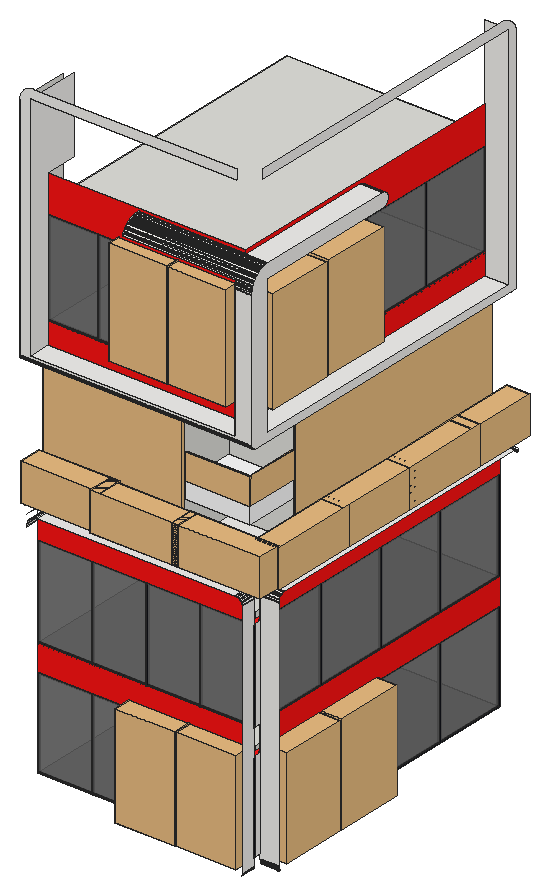
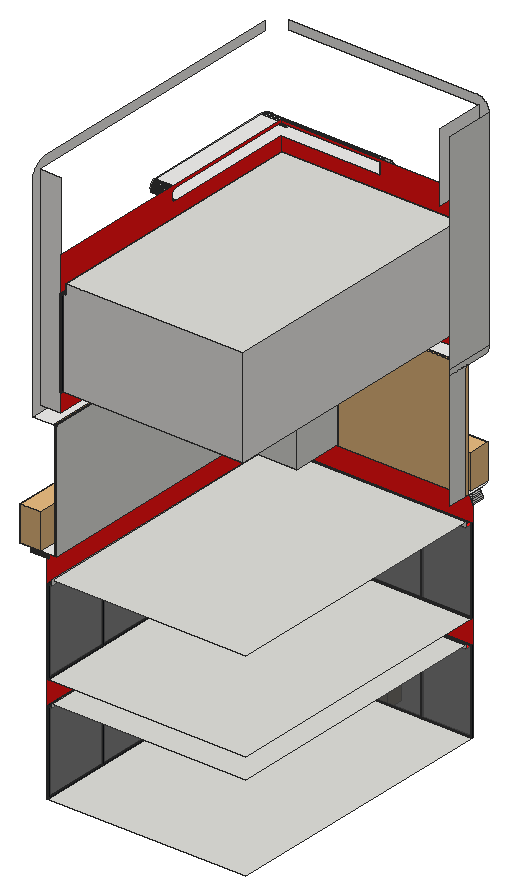
# SketchUp Ruby script. Lengths in inches.
U = 1.inch
M = Sketchup.active_model
def pt(a) = Geom::Point3d.new(a.map { |v| v * U })
def face(e, loops, mat)
  f = e.add_face(loops[0].map { |a| pt(a) })
  loops[1..].each { |l| e.add_face(l.map { |a| pt(a) }).erase! }
  f.material = f.back_material = mat if mat
  f
end
# faces: each face lists its corners as indices into pts; further lists are holes
def faces(e, pts, list, mat = nil) = list.each { |f| face(e, (f[0].is_a?(Array) ? f : [f]).map { |l| l.map { |i| pts[i] } }, mat) }
# xy, xz, yz: faces in a plane at the given z, y or x. An outline is a flat list of corners, or four numbers for a rectangle; further outlines are holes
def ring(l) = l.size == 4 ? [[l[0], l[1]], [l[2], l[1]], [l[2], l[3]], [l[0], l[3]]] : l.each_slice(2).to_a
def flat(e, list, mat, &to3) = list.each { |f| face(e, (f[0].is_a?(Array) ? f : [f]).map { |l| ring(l).map { |u, v| to3.(u, v) } }, mat) }
def xy(e, z, list, mat = nil) = flat(e, list, mat) { |x, y| [x, y, z] }
def xz(e, y, list, mat = nil) = flat(e, list, mat) { |x, z| [x, y, z] }
def yz(e, x, list, mat = nil) = flat(e, list, mat) { |y, z| [x, y, z] }
def lines(e, pts, list) = list.each { |a, b| e.add_line(pt(pts[a]), pt(pts[b])) }
# prism: a flat outline (further loops are holes) pulled along v
def prism(e, loops, v, mat = nil)
  f = face(e, loops, mat); d = Geom::Vector3d.new(v.map { |x| x * U })
  f.pushpull(f.normal.samedirection?(d) ? d.length : -d.length)
end
def box(e, o, s, mat = nil) = prism(e, [[o, [o[0] + s[0], o[1], o[2]], [o[0] + s[0], o[1] + s[1], o[2]], [o[0], o[1] + s[1], o[2]]]], [0, 0, s[2]], mat)
def at(x, y, z, deg = 0) = Geom::Transformation.translation(pt([x, y, z])) * Geom::Transformation.rotation(ORIGIN, Z_AXIS, deg.degrees)
def axes(o, x, y, z) = Geom::Transformation.new([*x, 0, *y, 0, *z, 0, *pt(o).to_a, 1])
def part(name) = M.definitions.add(name)
# library, detail: a bought-in or finely detailed component or shape, given as its bounding box
def library(name, o, s) = part(name).tap { |d| box(d.entities, o, s) }
def detail(e, o, s) = box(e.add_group.entities, o, s)
def put(e, d, t, mat = nil) = e.add_instance(d, t).tap { |i| i.material = mat if mat }
def group(e, t, mat = nil) = e.add_group.tap { |g| g.transformation = t; g.material = mat if mat }.entities
root = M.entities
M.materials.add("Generic").color = [242, 241, 238]
M.materials.add("Heather_Band").color = [255, 20, 20]
M.materials.add("[Color M00]").color = [255, 255, 255]
M.materials.add("{045efeae-c101-a24d-bd9b-6f5600100adb}").color = [102, 102, 102]
M.materials["{045efeae-c101-a24d-bd9b-6f5600100adb}"].alpha = 0.7
M.materials.add("{16756a1b-d383-d94f-ad82-104813d2624f}").color = [19, 21, 27]
c1 = library("Shrub+_Grass",[-121.83,-22.34,0],[123.96,19.94,123.95])
c2 = part("Furniture_0DcpanrIvuI8n_9Ae92L5A")
g1 = group(c2.entities,at(0,0,0))
box(g1,[-19.29,-0.2,0.39],[38.58,0.4,83.86],"{045efeae-c101-a24d-bd9b-6f5600100adb}")
g2 = group(c2.entities,at(0,0,0))
box(g2,[-19.68,-0.59,63.39],[39.36,1.18,0.39],"{16756a1b-d383-d94f-ad82-104813d2624f}")
box(g2,[-19.68,-0.59,42.52],[39.36,1.18,0.39],"{16756a1b-d383-d94f-ad82-104813d2624f}")
box(g2,[-19.68,-0.59,21.26],[39.36,1.18,0.39],"{16756a1b-d383-d94f-ad82-104813d2624f}")
xy(g2,0,[[-19.68,-0.59,19.68,0.59]],"{16756a1b-d383-d94f-ad82-104813d2624f}")
xy(g2,0.39,[[-19.68,-0.59,-19.29,0.59],[-19.68,-0.59,19.68,0.59],[19.29,-0.59,19.68,0.59]],"{16756a1b-d383-d94f-ad82-104813d2624f}")
xy(g2,84.25,[[-19.68,-0.59,19.68,0.59]],"{16756a1b-d383-d94f-ad82-104813d2624f}")
xy(g2,84.65,[[-19.68,-0.59,-19.29,0.59],[-19.68,-0.59,19.68,0.59],[19.29,-0.59,19.68,0.59]],"{16756a1b-d383-d94f-ad82-104813d2624f}")
xz(g2,-0.59,[[-19.68,0,19.68,0.39],[-19.68,0.39,-19.29,84.65],[19.29,0.39,19.68,84.65],[-19.68,84.25,19.68,84.65]],"{16756a1b-d383-d94f-ad82-104813d2624f}")
xz(g2,0.59,[[-19.68,0,19.68,0.39],[-19.68,0.39,-19.29,84.65],[19.29,0.39,19.68,84.65],[-19.68,84.25,19.68,84.65]],"{16756a1b-d383-d94f-ad82-104813d2624f}")
yz(g2,-19.68,[[-0.59,0,0.59,0.39],[-0.59,0.39,0.59,84.65],[-0.59,84.25,0.59,84.65]],"{16756a1b-d383-d94f-ad82-104813d2624f}")
yz(g2,-19.29,[[-0.59,0.39,0.59,84.65]],"{16756a1b-d383-d94f-ad82-104813d2624f}")
yz(g2,19.29,[[-0.59,0.39,0.59,84.65]],"{16756a1b-d383-d94f-ad82-104813d2624f}")
yz(g2,19.68,[[-0.59,0,0.59,0.39],[-0.59,0.39,0.59,84.65],[-0.59,84.25,0.59,84.65]],"{16756a1b-d383-d94f-ad82-104813d2624f}")
c3 = part("Glass+Window")
put(c3.entities,c2,at(0,0,-42.32))
c4 = library("Back Drop",[0,0,0],[82.68,2.27,107.48])
c5 = library("Planted timber trough",[0,0,0],[56.02,15.3,25.28])
c6 = library("My+Glass_Railing",[-0.07,0,0],[101.37,2.52,40.9])
c7 = library("My+Glass_Railing\#1",[-0.0625,0,0],[98.32,2.52,40.9])
xy(root,452.24,[[145.77,137.375,482.71,617.58]])
xy(root,592.96,[[145.77,137.375,145.77,151.79,474.55,151.79,474.55,617.58,482.71,617.58,482.71,137.375]],"Heather_Band")
xy(root,599,[[145.77,151.79,474.55,617.58]])
xy(root,633.64,[[145.77,137.375,482.71,617.58]])
xy(root,777.77,[[145.77,137.375,145.77,151.79,474.55,151.79,474.55,617.58,482.71,617.58,482.71,137.375]],"Heather_Band")
xy(root,786.62,[[145.77,151.79,474.55,617.58]])
xy(root,823.39,[[480.21,611.74,482.71,617.58]])
xy(root,823.39,[[164.14,115.9,470.91,137.375],[482.71,163.53,510.83,611.74]],"Generic")
xy(root,835.52,[[144.5,115.9,492.12,115.9,494.5625,116.0625,496.96,116.54,499.28,117.33,501.48,118.41,503.51,119.77,505.35,121.38,506.97,123.22,508.33,125.26,509.41,127.45,510.2,129.77,510.67,132.17,510.83,134.62,510.83,624.64,510.77,625.65,510.57,626.63,510.25,627.59,509.8,628.49,509.24,629.33,508.58,630.08,507.82,630.75,506.98,631.31,506.08,631.75,505.13,632.08,504.14,632.27,503.14,632.34,454.94,632.34,454.94,249.57,353.58,249.57,353.58,164.53,133.86,164.53,133.86,126.54,133.95,125.15,134.22,123.79,134.67,122.47,135.28,121.22,136.06,120.0625,136.98,119.02,138.02,118.1,139.18,117.33,140.43,116.71,141.75,116.26,143.11,115.99]],"Generic")
xy(root,895.84,[[353.58,164.53,454.94,249.57]],"[Color M00]")
xy(root,921.04,[[353.58,164.53,454.94,164.53,454.94,249.57,449.01,249.57,449.01,170.19,353.58,170.19]],"Generic")
xy(root,921.04,[[353.58,170.19,449.01,249.57]],"[Color M00]")
xy(root,1033.75,[[133.86,124.82,133.86,164.53,353.58,164.53,353.58,249.57,454.94,249.57,454.94,632.34,486.44,632.34,487.65,632.26,488.84,632.02,489.98,631.63,491.07,631.1,492.08,630.43,492.99,629.625,493.79,628.72,494.46,627.71,495,626.62,495.38,625.48,495.62,624.29,495.7,623.08,495.7,124.82],[495.7,623.08,495.62,624.29,495.38,625.48,495,626.62,494.46,627.71,493.79,628.72,492.99,629.625,492.08,630.43,491.07,631.1,489.98,631.63,488.84,632.02,487.65,632.26,486.44,632.34,495.7,632.34]],"Generic")
xy(root,1045.51,[[150.95,118.26,469.09,118.26,469.09,128.11,487.7,128.11,487.7,146.81,495.7,146.81,495.7,617.58,459.56,617.58,459.56,151.96,150.95,151.96]],"Generic")
xy(root,1078.9375,[[150.95,151.96,459.56,617.58]])
xy(root,1227.79,[[150.95,151.96,150.95,160.3,451.22,160.3,451.22,617.58,459.56,617.58,459.56,151.96]],"Heather_Band")
xy(root,1245.125,[[150.95,160.3,451.22,617.58]])
xy(root,1261.55,[[291.94,120.41,291.94,151.96,459.56,151.96,459.56,372.87,495.7,372.87,495.7,146.81,487.7,146.81,487.7,128.11,469.09,128.11,469.09,120.41]],"Generic")
xy(root,1281.6,[[291.94,149.74,495.7,149.74,495.7,372.87,459.56,372.87,459.56,151.96,291.94,151.96]],"Generic")
xz(root,118.26,[[133.86,1040.31,495.7,1040.31,495.7,1250.12,469.09,1250.12,469.09,1045.51,150.95,1045.51,150.95,1403.29,472.44,1403.29,472.44,1418.32,155.71,1418.32,154.28,1418.27,152.86,1418.13,151.45,1417.9,150.06,1417.57,148.6875,1417.16,147.35,1416.65,146.05,1416.0625,144.79,1415.39,143.57,1414.63,142.41,1413.8,141.3,1412.89,140.26,1411.92,139.28,1410.875,138.375,1409.77,137.54,1408.61,136.79,1407.39,136.11,1406.13,135.52,1404.83,135.02,1403.49,134.6,1402.12,134.28,1400.73,134.05,1399.32,133.91,1397.89,133.86,1396.46]],"Generic")
xz(root,128.11,[[469.09,1045.51,487.7,1261.55]])
xz(root,137.375,[[145.77,592.96,482.71,633.64],[145.77,777.77,482.71,777.77,482.71,812.85,482.46,814.27,482.04,815.65,481.46,816.97,480.72,818.21,479.84,819.35,478.82,820.37,477.69,821.27,476.46,822.02,475.14,822.61,473.77,823.04,472.35,823.3,470.91,823.39,164.14,823.39,161.74,823.23,159.38,822.77,157.11,821.99,154.95,820.93,152.95,819.6,151.15,818.01,149.5625,816.21,148.23,814.21,147.17,812.05,146.39,809.78,145.93,807.42,145.77,805.02]],"Heather_Band")
xz(root,146.81,[[487.7,1045.51,495.7,1261.55]])
xz(root,150.43,[[482.71,444.64,510.83,812.2]],"Generic")
xz(root,151.79,[[145.77,592.96,474.55,599],[145.77,777.77,474.55,786.62]])
xz(root,151.96,[[150.95,1045.51,459.56,1078.9375],[150.95,1227.79,459.56,1227.79,459.56,1261.55,291.94,1261.55,291.94,1281.6,459.56,1281.6,459.56,1286.04,150.95,1286.04]],"Heather_Band")
xz(root,160.3,[[150.95,1227.79,451.22,1245.125]])
xz(root,164.53,[[133.86,835.52,353.58,1033.75]])
xz(root,164.53,[[353.58,895.84,454.94,921.04]],"[Color M00]")
xz(root,249.57,[[353.58,835.52,454.94,895.84],[353.58,921.04,454.94,1033.75]])
xz(root,617.58,[[480.21,817.55,482.71,823.39]])
xz(root,617.58,[[459.56,1045.51,495.7,1045.51,495.7,1403.29,459.56,1403.29,459.56,1227.79,451.22,1227.79,451.22,1245.125,150.95,1245.125,150.95,1078.9375,459.56,1078.9375]],"Generic")
yz(root,133.86,[[164.53,835.52,200.9,1033.75],[124.82,1033.75,123.96,1033.8,123.12,1033.97,122.31,1034.25,121.54,1034.63,120.82,1035.1,120.18,1035.67,119.61,1036.31,119.14,1037.03,118.76,1037.8,118.48,1038.61,118.3125,1039.45,118.26,1040.31,118.26,1042.88,200.9,1042.88,200.9,1033.75],[118.26,1042.88,200.9,1396.46]])
yz(root,150.95,[[118.26,1045.51,151.96,1045.51,151.96,1078.9375,617.58,1078.9375,617.58,1245.125,160.3,1245.125,160.3,1227.79,151.96,1227.79,151.96,1286.04,200.9,1286.04,200.9,1403.29,118.26,1403.29]],"Generic")
yz(root,291.94,[[120.41,1261.55,120.98,1262.92,121.69,1264.41,122.48,1265.86,123.34,1267.27,124.27,1268.625,125.27,1269.93,126.34,1271.18,127.48,1272.38,128.68,1273.52,129.93,1274.59,131.24,1275.59,132.59,1276.52,134,1277.38,135.45,1278.17,136.9375,1278.88,138.46,1279.51,140.01,1280.0625,141.59,1280.53,143.2,1280.91,144.82,1281.21,146.45,1281.43,148.09,1281.56,149.74,1281.6,151.96,1281.6,151.96,1261.55]])
yz(root,353.58,[[164.53,835.52,249.57,895.84],[164.53,921.04,249.57,1033.75]])
yz(root,451.22,[[160.3,1227.79,617.58,1245.125]])
yz(root,454.94,[[249.57,835.52,632.34,1033.75]])
yz(root,454.94,[[164.53,895.84,249.57,921.04]],"[Color M00]")
yz(root,459.56,[[151.96,1045.51,617.58,1078.9375],[151.96,1227.79,617.58,1227.79,617.58,1286.04,151.96,1286.04,151.96,1281.6,372.87,1281.6,373.91,1281.55,374.95,1281.38,375.96,1281.11,376.94,1280.74,377.88,1280.26,378.76,1279.6875,379.57,1279.03,380.32,1278.29,380.98,1277.47,381.55,1276.59,382.02,1275.66,382.4,1274.68,382.67,1273.66,382.84,1272.625,382.89,1271.58,382.84,1270.53,382.67,1269.49,382.4,1268.48,382.02,1267.5,381.55,1266.57,380.98,1265.6875,380.32,1264.87,379.57,1264.13,378.76,1263.47,377.88,1262.9,376.94,1262.42,375.96,1262.04,374.95,1261.77,373.91,1261.61,372.87,1261.55,151.96,1261.55]],"Heather_Band")
yz(root,469.09,[[118.26,1045.51,118.26,1250.12,118.3,1251.77,118.43,1253.41,118.65,1255.04,118.95,1256.66,119.33,1258.27,119.8,1259.85,120.35,1261.4,120.41,1261.55,128.11,1261.55,128.11,1045.51]])
yz(root,474.55,[[151.79,592.96,617.58,599],[151.79,777.77,617.58,786.62]])
yz(root,480.21,[[617.58,817.55,617.53,818.3125,617.39,819.0625,617.14,819.79,616.8,820.47,616.38,821.11,615.875,821.68,615.3,822.18,614.66,822.61,613.98,822.95,613.26,823.19,612.51,823.34,611.74,823.39,617.58,823.39]])
yz(root,482.71,[[115.9,439.07,115.9,812.85,137.375,812.85,137.375,777.77,150.43,777.77,150.43,633.64,137.375,633.64,137.375,592.96,150.43,592.96,150.43,452.24,137.375,452.24,137.375,439.07]],"Generic")
yz(root,482.71,[[150.43,592.96,617.58,633.64],[150.43,777.77,617.58,777.77,617.58,823.39,163.53,823.39,161.6,823.25,159.72,822.83,157.92,822.15,156.23,821.21,154.7,820.04,153.35,818.65,152.22,817.09,151.33,815.38,150.69,813.56,150.43,812.2]],"Heather_Band")
yz(root,487.7,[[128.11,1045.51,146.81,1261.55]])
yz(root,495.7,[[124.82,1033.75,632.34,1033.75,632.34,1395.5,631.92,1397.1,631.4,1398.67,630.81,1400.21,630.125,1401.71,629.36,1403.18,628.51,1404.59,627.59,1405.96,626.59,1407.28,625.52,1408.54,624.38,1409.73,623.18,1410.86,621.91,1411.92,620.59,1412.91,619.21,1413.83,617.79,1414.66,616.32,1415.42,614.81,1416.09,613.27,1416.67,611.69,1417.17,610.09,1417.58,608.47,1417.9,606.84,1418.13,605.19,1418.27,603.54,1418.32,139.65,1418.32,139.65,1403.29,617.58,1403.29,617.58,1045.51,146.81,1045.51,146.81,1261.55,372.87,1261.55,373.91,1261.61,374.95,1261.77,375.96,1262.04,376.94,1262.42,377.88,1262.9,378.76,1263.47,379.57,1264.13,380.32,1264.87,380.98,1265.6875,381.55,1266.57,382.02,1267.5,382.4,1268.48,382.67,1269.49,382.84,1270.53,382.89,1271.58,382.84,1272.625,382.67,1273.66,382.4,1274.68,382.02,1275.66,381.55,1276.59,380.98,1277.47,380.32,1278.29,379.57,1279.03,378.76,1279.6875,377.88,1280.26,376.94,1280.74,375.96,1281.11,374.95,1281.38,373.91,1281.55,372.87,1281.6,149.74,1281.6,148.09,1281.56,146.45,1281.43,144.82,1281.21,143.2,1280.91,141.59,1280.53,140.01,1280.0625,138.46,1279.51,136.9375,1278.88,135.45,1278.17,134,1277.38,132.59,1276.52,131.24,1275.59,129.93,1274.59,128.68,1273.52,127.48,1272.38,126.34,1271.18,125.27,1269.93,124.27,1268.625,123.34,1267.27,122.48,1265.86,121.69,1264.41,120.98,1262.92,120.35,1261.4,119.8,1259.85,119.33,1258.27,118.95,1256.66,118.65,1255.04,118.43,1253.41,118.3,1251.77,118.26,1250.12,118.26,1040.31,118.3125,1039.45,118.48,1038.61,118.76,1037.8,119.14,1037.03,119.61,1036.31,120.18,1035.67,120.82,1035.1,121.54,1034.63,122.31,1034.25,123.12,1033.97,123.96,1033.8]],"Generic")
p = [[510.83,153.22,436.74],[510.83,154.17,435.68],[482.71,154.17,435.68],[482.71,153.22,436.74],[482.01,115.9,436.03],[482.4,115.9,437],
  [482.4,137.375,437],[482.01,137.375,436.03],[510.83,152.39,437.89],[482.71,152.39,437.89],[482.63,115.9,438.03],[482.63,137.375,438.03],
  [510.83,151.69,439.14],[482.71,151.69,439.14],[482.71,115.9,439.07],[482.71,137.375,439.07],[510.83,151.15,440.45],[482.71,151.15,440.45],
  [510.83,150.75,441.82],[482.71,150.75,441.82],[510.83,150.51,443.22],[482.71,150.51,443.22],[510.83,150.43,444.64],[482.71,150.43,444.64],
  [145.93,115.9,807.42],[145.77,115.9,805.02],[145.77,137.375,805.02],[145.93,137.375,807.42],[146.39,115.9,809.78],[146.39,137.375,809.78],
  [147.17,115.9,812.05],[147.17,137.375,812.05],[148.23,115.9,814.21],[148.23,137.375,814.21],[510.83,150.69,813.56],[510.83,150.43,812.2],
  [482.71,150.43,812.2],[482.71,150.69,813.56],[482.71,115.9,812.85],[482.46,115.9,814.27],[482.46,137.375,814.27],[482.71,137.375,812.85],
  [510.83,151.33,815.38],[482.71,151.33,815.38],[149.5625,115.9,816.21],[149.5625,137.375,816.21],[482.04,115.9,815.65],[482.04,137.375,815.65],
  [510.83,152.22,817.09],[482.71,152.22,817.09],[481.46,115.9,816.97],[481.46,137.375,816.97],[151.15,115.9,818.01],[151.15,137.375,818.01],
  [480.72,115.9,818.21],[480.72,137.375,818.21],[510.83,153.35,818.65],[482.71,153.35,818.65],[510.83,617.58,817.55],[510.83,617.53,818.3125],
  [480.21,617.53,818.3125],[480.21,617.58,817.55],[482.71,617.58,817.55],[152.95,115.9,819.6],[152.95,137.375,819.6],[479.84,115.9,819.35],
  [479.84,137.375,819.35],[510.83,617.39,819.0625],[480.21,617.39,819.0625],[510.83,154.7,820.04],[482.71,154.7,820.04],[510.83,617.14,819.79],
  [480.21,617.14,819.79],[478.82,115.9,820.37],[478.82,137.375,820.37],[154.95,115.9,820.93],[154.95,137.375,820.93],[510.83,616.8,820.47],
  [480.21,616.8,820.47],[510.83,156.23,821.21],[482.71,156.23,821.21],[477.69,115.9,821.27],[477.69,137.375,821.27],[510.83,616.38,821.11],
  [480.21,616.38,821.11],[157.11,115.9,821.99],[157.11,137.375,821.99],[510.83,615.875,821.68],[480.21,615.875,821.68],[510.83,157.92,822.15],
  [482.71,157.92,822.15],[476.46,115.9,822.02],[476.46,137.375,822.02],[510.83,615.3,822.18],[480.21,615.3,822.18],[159.38,115.9,822.77],
  [159.38,137.375,822.77],[475.14,115.9,822.61],[475.14,137.375,822.61],[510.83,159.72,822.83],[482.71,159.72,822.83],[510.83,614.66,822.61],
  [480.21,614.66,822.61],[473.77,115.9,823.04],[473.77,137.375,823.04],[510.83,613.98,822.95],[480.21,613.98,822.95],[161.74,115.9,823.23],
  [161.74,137.375,823.23],[510.83,161.6,823.25],[482.71,161.6,823.25],[510.83,613.26,823.19],[480.21,613.26,823.19],[472.35,115.9,823.3],
  [472.35,137.375,823.3],[164.14,115.9,823.39],[164.14,137.375,823.39],[510.83,612.51,823.34],[480.21,612.51,823.34],[470.91,115.9,823.39],
  [470.91,137.375,823.39],[510.83,163.53,823.39],[482.71,163.53,823.39],[510.83,611.74,823.39],[482.71,611.74,823.39],[480.21,611.74,823.39],
  [495.7,124.82,1033.75],[495.7,123.96,1033.8],[133.86,123.96,1033.8],[133.86,124.82,1033.75],[495.7,123.12,1033.97],[133.86,123.12,1033.97],
  [495.7,122.31,1034.25],[133.86,122.31,1034.25],[495.7,121.54,1034.63],[133.86,121.54,1034.63],[495.7,120.82,1035.1],[133.86,120.82,1035.1],
  [495.7,120.18,1035.67],[133.86,120.18,1035.67],[495.7,119.61,1036.31],[133.86,119.61,1036.31],[495.7,119.14,1037.03],[133.86,119.14,1037.03],
  [495.7,118.76,1037.8],[133.86,118.76,1037.8],[495.7,118.48,1038.61],[133.86,118.48,1038.61],[495.7,118.3125,1039.45],[133.86,118.3125,1039.45],
  [495.7,118.26,1040.31],[133.86,118.26,1040.31],[495.7,118.26,1250.12],[495.7,118.3,1251.77],[469.09,118.3,1251.77],[469.09,118.26,1250.12],
  [495.7,118.43,1253.41],[469.09,118.43,1253.41],[495.7,118.65,1255.04],[469.09,118.65,1255.04],[495.7,118.95,1256.66],[469.09,118.95,1256.66],
  [495.7,119.33,1258.27],[469.09,119.33,1258.27],[495.7,119.8,1259.85],[469.09,119.8,1259.85],[495.7,120.35,1261.4],[469.09,120.35,1261.4],
  [495.7,120.98,1262.92],[291.94,120.98,1262.92],[291.94,120.41,1261.55],[469.09,120.41,1261.55],[495.7,373.91,1261.61],[495.7,372.87,1261.55],
  [459.56,372.87,1261.55],[459.56,373.91,1261.61],[495.7,374.95,1261.77],[459.56,374.95,1261.77],[495.7,375.96,1262.04],[459.56,375.96,1262.04],
  [495.7,376.94,1262.42],[459.56,376.94,1262.42],[495.7,377.88,1262.9],[459.56,377.88,1262.9],[495.7,121.69,1264.41],[291.94,121.69,1264.41],
  [495.7,378.76,1263.47],[459.56,378.76,1263.47],[495.7,379.57,1264.13],[459.56,379.57,1264.13],[495.7,380.32,1264.87],[459.56,380.32,1264.87],
  [495.7,122.48,1265.86],[291.94,122.48,1265.86],[495.7,380.98,1265.6875],[459.56,380.98,1265.6875],[495.7,381.55,1266.57],[459.56,381.55,1266.57],
  [495.7,123.34,1267.27],[291.94,123.34,1267.27],[495.7,382.02,1267.5],[459.56,382.02,1267.5],[495.7,124.27,1268.625],[291.94,124.27,1268.625],
  [495.7,382.4,1268.48],[459.56,382.4,1268.48],[495.7,382.67,1269.49],[459.56,382.67,1269.49],[495.7,125.27,1269.93],[291.94,125.27,1269.93],
  [495.7,382.84,1270.53],[459.56,382.84,1270.53],[495.7,126.34,1271.18],[291.94,126.34,1271.18],[495.7,382.89,1271.58],[459.56,382.89,1271.58],
  [495.7,127.48,1272.38],[291.94,127.48,1272.38],[495.7,382.84,1272.625],[459.56,382.84,1272.625],[495.7,128.68,1273.52],[291.94,128.68,1273.52],
  [495.7,382.67,1273.66],[459.56,382.67,1273.66],[495.7,129.93,1274.59],[291.94,129.93,1274.59],[495.7,382.4,1274.68],[459.56,382.4,1274.68],
  [495.7,131.24,1275.59],[291.94,131.24,1275.59],[495.7,382.02,1275.66],[459.56,382.02,1275.66],[495.7,132.59,1276.52],[291.94,132.59,1276.52],
  [495.7,381.55,1276.59],[459.56,381.55,1276.59],[495.7,134,1277.38],[291.94,134,1277.38],[495.7,380.98,1277.47],[459.56,380.98,1277.47],
  [495.7,135.45,1278.17],[291.94,135.45,1278.17],[495.7,380.32,1278.29],[459.56,380.32,1278.29],[495.7,136.9375,1278.88],[291.94,136.9375,1278.88],
  [495.7,379.57,1279.03],[459.56,379.57,1279.03],[495.7,138.46,1279.51],[291.94,138.46,1279.51],[495.7,378.76,1279.6875],[459.56,378.76,1279.6875],
  [495.7,140.01,1280.0625],[291.94,140.01,1280.0625],[495.7,377.88,1280.26],[459.56,377.88,1280.26],[495.7,141.59,1280.53],[291.94,141.59,1280.53],
  [495.7,376.94,1280.74],[459.56,376.94,1280.74],[495.7,143.2,1280.91],[291.94,143.2,1280.91],[495.7,375.96,1281.11],[459.56,375.96,1281.11],
  [495.7,144.82,1281.21],[291.94,144.82,1281.21],[495.7,374.95,1281.38],[459.56,374.95,1281.38],[495.7,146.45,1281.43],[291.94,146.45,1281.43],
  [495.7,148.09,1281.56],[291.94,148.09,1281.56],[495.7,373.91,1281.55],[459.56,373.91,1281.55],[495.7,372.87,1281.6],[459.56,372.87,1281.6],
  [495.7,149.74,1281.6],[291.94,149.74,1281.6],[482.71,150.43,823.39],[145.77,137.375,823.39],[451.61,151.96,1072.125],[451.61,159.91,1072.125],
  [482.71,137.375,823.39],[469.09,118.26,1261.55],[510.83,617.58,823.39],[482.71,617.58,823.39],[510.83,150.43,823.39],[145.77,115.9,823.39],
  [482.71,115.9,823.39]]
faces(root,p,[[0,1,2,3],[4,5,6,7],[8,0,3,9],[5,10,11,6],[12,8,9,13],[10,14,15,11],[16,12,13,17],[18,16,17,19],
  [20,18,19,21],[22,20,21,23],[24,25,26,27],[28,24,27,29],[30,28,29,31],[32,30,31,33],[34,35,36,37],[38,39,40,41],
  [42,34,37,43],[44,32,33,45],[39,46,47,40],[48,42,43,49],[46,50,51,47],[52,44,45,53],[50,54,55,51],[56,48,49,57],
  [58,59,60,61,62],[63,52,53,64],[54,65,66,55],[59,67,68,60],[69,56,57,70],[67,71,72,68],[65,73,74,66],[75,63,64,76],
  [71,77,78,72],[79,69,70,80],[73,81,82,74],[77,83,84,78],[85,75,76,86],[83,87,88,84],[89,79,80,90],[81,91,92,82],
  [87,93,94,88],[95,85,86,96],[91,97,98,92],[99,89,90,100],[93,101,102,94],[97,103,104,98],[101,105,106,102],[107,95,96,108],
  [109,99,100,110],[105,111,112,106],[103,113,114,104],[115,107,108,116],[111,117,118,112],[113,119,120,114],[121,109,110,122],[117,123,124,125,118],
  [126,127,128,129],[127,130,131,128],[130,132,133,131],[132,134,135,133],[134,136,137,135],[136,138,139,137],[138,140,141,139],[140,142,143,141],
  [142,144,145,143],[144,146,147,145],[146,148,149,147],[148,150,151,149],[152,153,154,155],[153,156,157,154],[156,158,159,157],[158,160,161,159],
  [160,162,163,161],[162,164,165,163],[164,166,167,165],[166,168,169,170,171,167],[172,173,174,175],[176,172,175,177],[178,176,177,179],[180,178,179,181],
  [182,180,181,183],[168,184,185,169],[186,182,183,187],[188,186,187,189],[190,188,189,191],[184,192,193,185],[194,190,191,195],[196,194,195,197],
  [192,198,199,193],[200,196,197,201],[198,202,203,199],[204,200,201,205],[206,204,205,207],[202,208,209,203],[210,206,207,211],[208,212,213,209],
  [214,210,211,215],[212,216,217,213],[218,214,215,219],[216,220,221,217],[222,218,219,223],[220,224,225,221],[226,222,223,227],[224,228,229,225],
  [230,226,227,231],[228,232,233,229],[234,230,231,235],[232,236,237,233],[238,234,235,239],[236,240,241,237],[242,238,239,243],[240,244,245,241],
  [246,242,243,247],[244,248,249,245],[250,246,247,251],[248,252,253,249],[254,250,251,255],[252,256,257,253],[258,254,255,259],[256,260,261,257],
  [262,258,259,263],[260,264,265,261],[266,262,263,267],[264,268,269,265],[268,270,271,269],[272,266,267,273],[274,272,273,275],[270,276,277,271]],"Generic")
lines(root,p,[[278,122],[279,116],[279,26],[280,281],[282,41],[278,36],[155,283],[284,285],[286,278],[287,279],[288,282],[120,282]])
put(root,c1,axes([474.45,140.67,445.36],[0.74635,0,0],[0,1.37,0],[0,0,1.28357]))
put(root,c1,axes([379.85,140.67,445.36],[0.74635,0,0],[0,1.37,0],[0,0,1.28357]))
put(root,c1,axes([478.77,262.12,445.36],[0,0.83415,0],[-1.64,0,0],[0,0,1.24654]))
put(root,c1,axes([478.77,373.86,445.36],[0,0.85966,0],[-1.64,0,0],[0,0,1.24654]))
put(root,c3,axes([314.24,138.68,522.6],[0,0,-3.57428],[0,2.2,0],[3.98066,0,0]),"Heather_Band")
put(root,c3,axes([481.41,384.01,522.6],[0,0,-3.57428],[-2.2,0,0],[0,5.51897,0]),"Heather_Band")
put(root,c3,axes([481.41,384.01,705.71],[0,0,-3.66085],[-2.2,0,0],[0,5.51897,0]))
put(root,c3,axes([314.24,138.68,705.71],[0,0,-3.66085],[0,2.2,0],[3.98066,0,0]),"Heather_Band")
put(root,c4,axes([458.72,632.34,835.52],[0,0,2.41699],[-1.66,0,0],[0,-3.56125,0]))
put(root,c5,axes([376.03,111.43,835.52],[2.46,0,0],[0,2.35,0],[0,0,2.3275]))
put(root,c5,axes([516.98,142.89,835.52],[0,2.46,0],[-2.35,0,0],[0,0,2.3275]))
put(root,c5,axes([516.98,270.66,835.52],[0,2.46,0],[-2.35,0,0],[0,0,2.3275]))
put(root,c5,axes([516.98,398.42,835.52],[0,2.46,0],[-2.35,0,0],[0,0,2.3275]))
put(root,c5,axes([516.98,520.86,835.52],[0,1.99011,0],[-2.35,0,0],[0,0,2.3275]))
put(root,c5,axes([248.22,111.43,835.52],[2.46,0,0],[0,2.35,0],[0,0,2.3275]))
put(root,c5,axes([137.01,115.53,835.52],[2.2386,0,0],[0,2.35,0],[0,0,2.3275]))
put(root,c4,axes([352.03,161.79,835.52],[0,0,2.39762],[0,1.66,0],[-2.02992,0,0]))
put(root,c6,at(353.54,164.53,921.04))
put(root,c7,at(454.91,167.56,921.05,89.855))
put(root,c1,axes([442.18,155.11,1070.32],[0.73171,0,0],[0,1,0],[0,0,1.32208]))
put(root,c1,axes([349.43,155.11,1070.32],[0.73171,0,0],[0,1,0],[0,0,1.32208]))
put(root,c1,axes([455.17,260.75,1073.42],[0,0.83415,0],[-1.8285,0,0],[0,0,1.29591]))
put(root,c1,axes([455.17,372.49,1073.42],[0,0.85966,0],[-1.8285,0,0],[0,0,1.29591]))
put(root,c3,axes([304.76,153.26,1153.36],[0,0,-3.78094],[0,2.2,0],[3.65763,0,0]),"Heather_Band")
put(root,c3,axes([458.26,386.18,1153.36],[0,0,-3.78094],[-2.2,0,0],[0,5.51897,0]),"Heather_Band")
